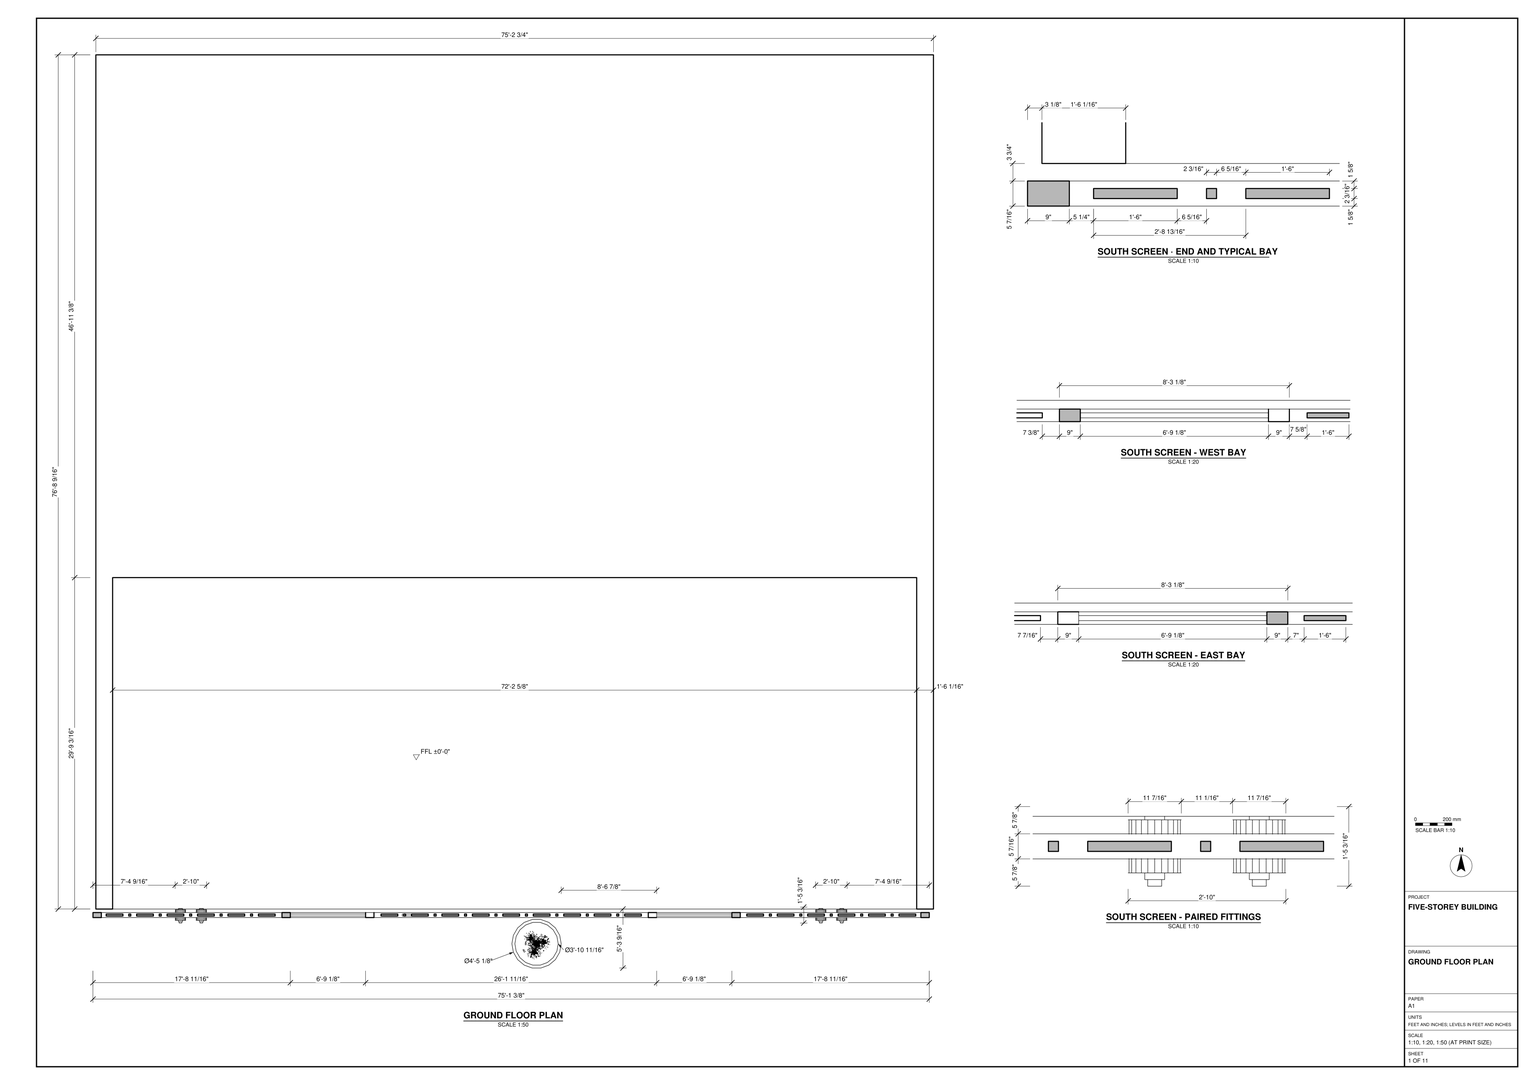
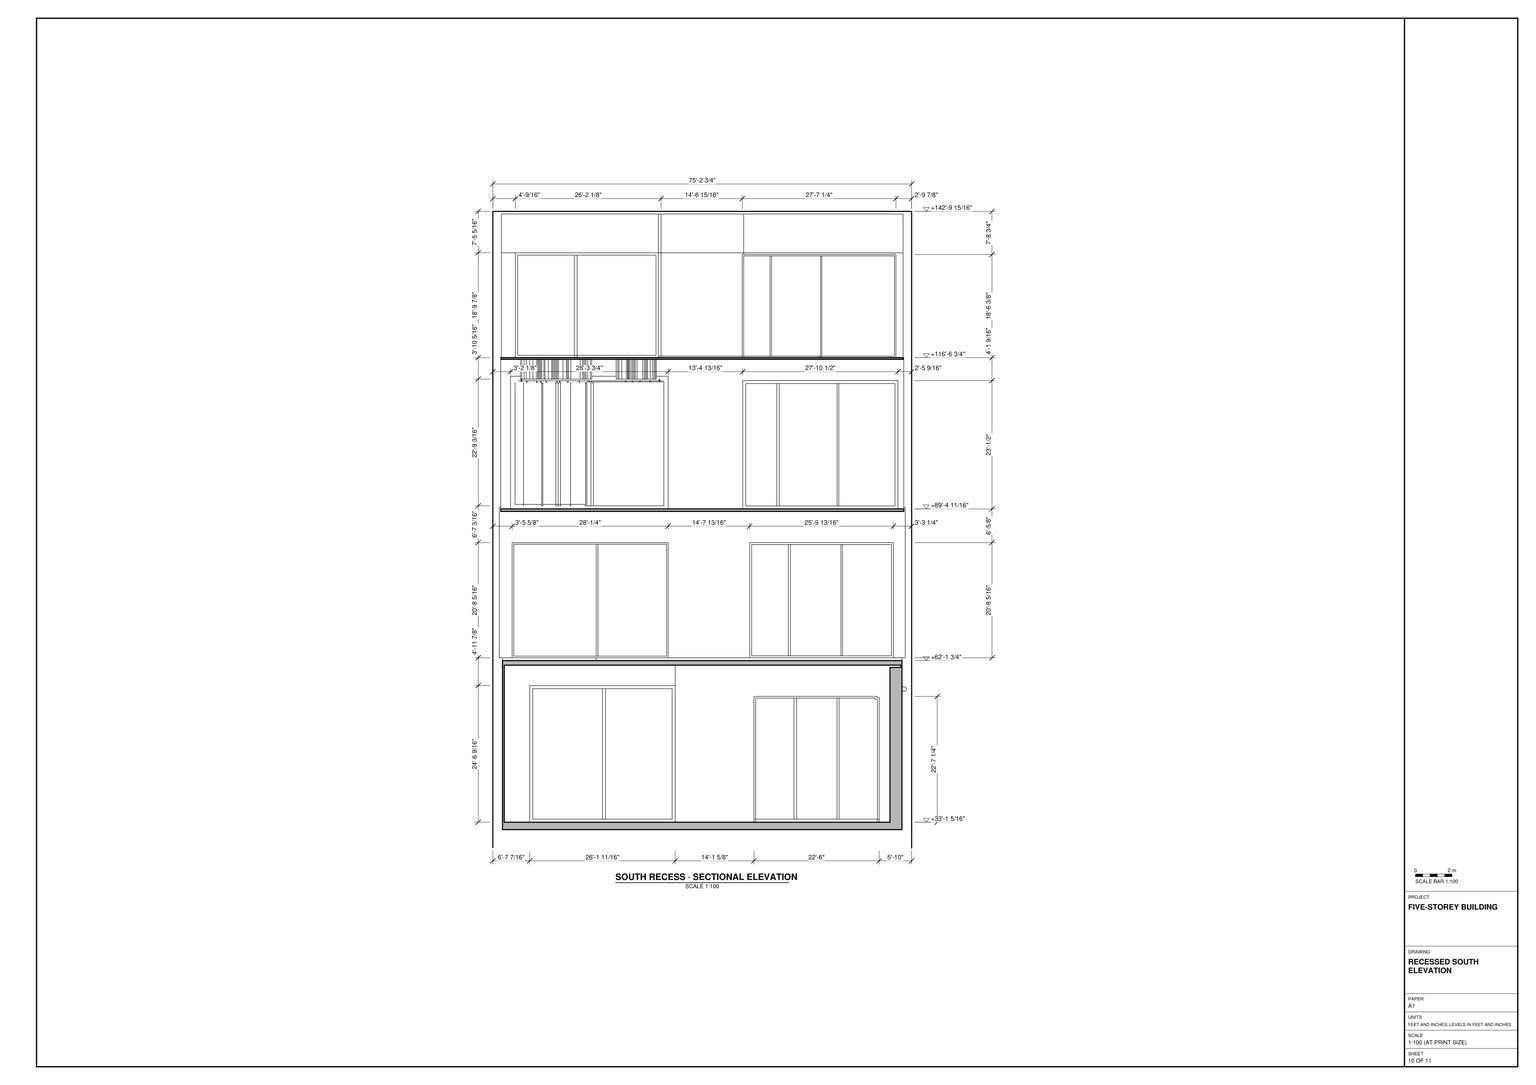
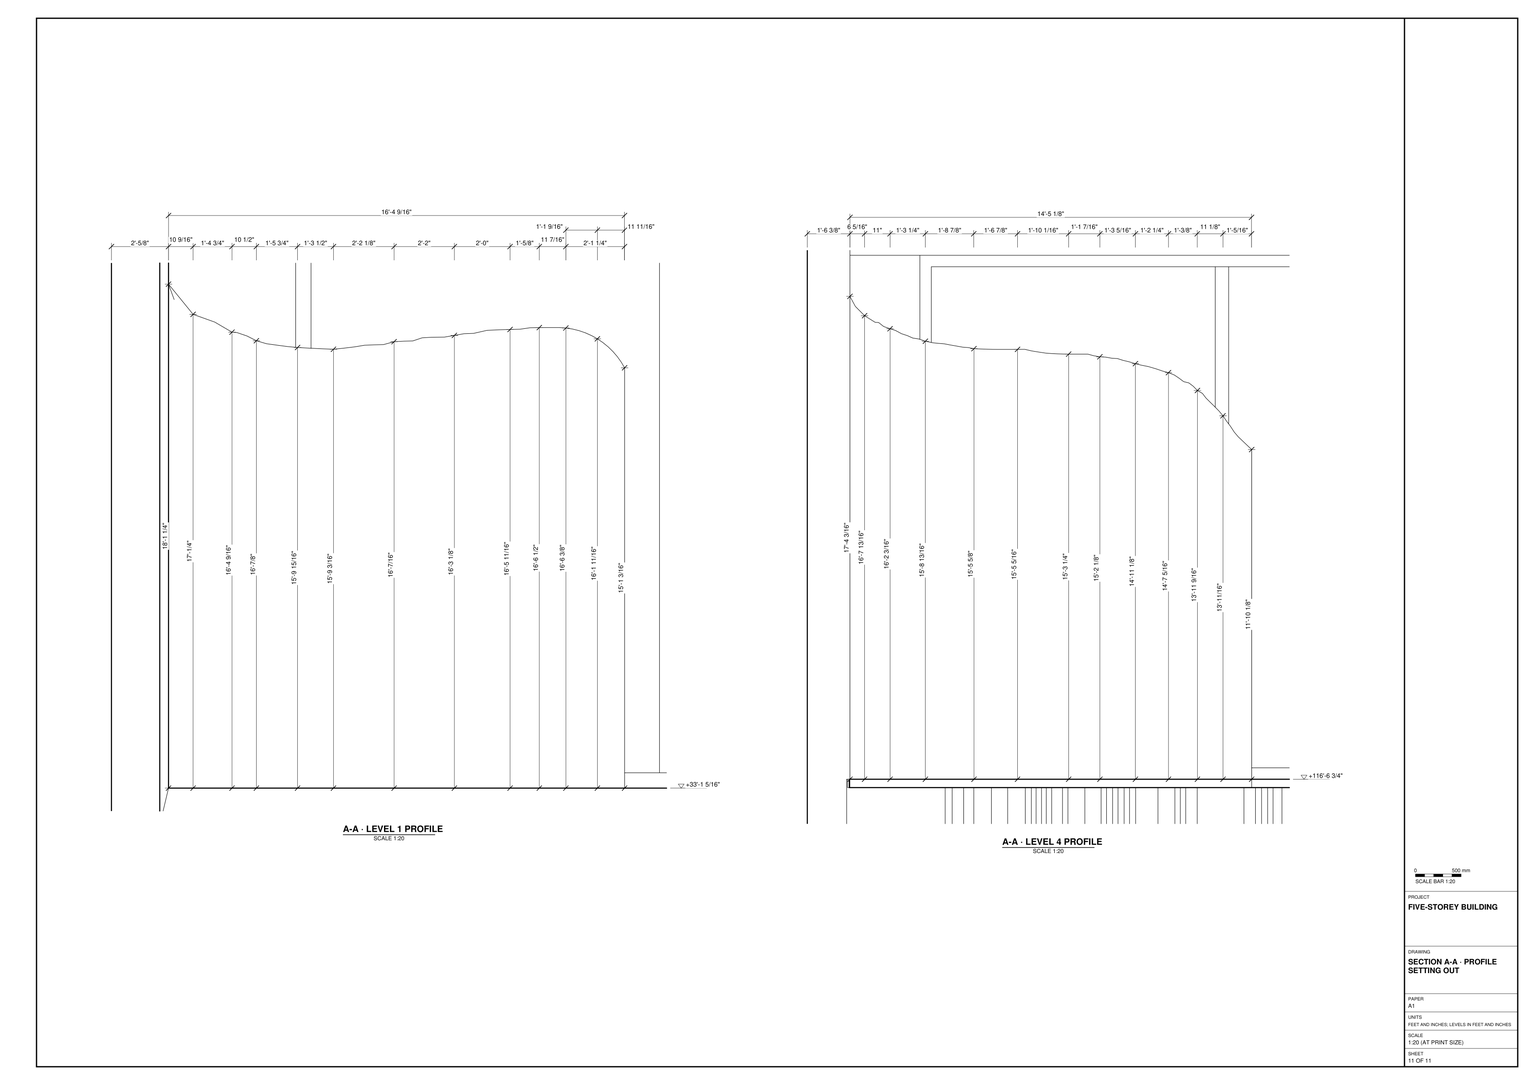
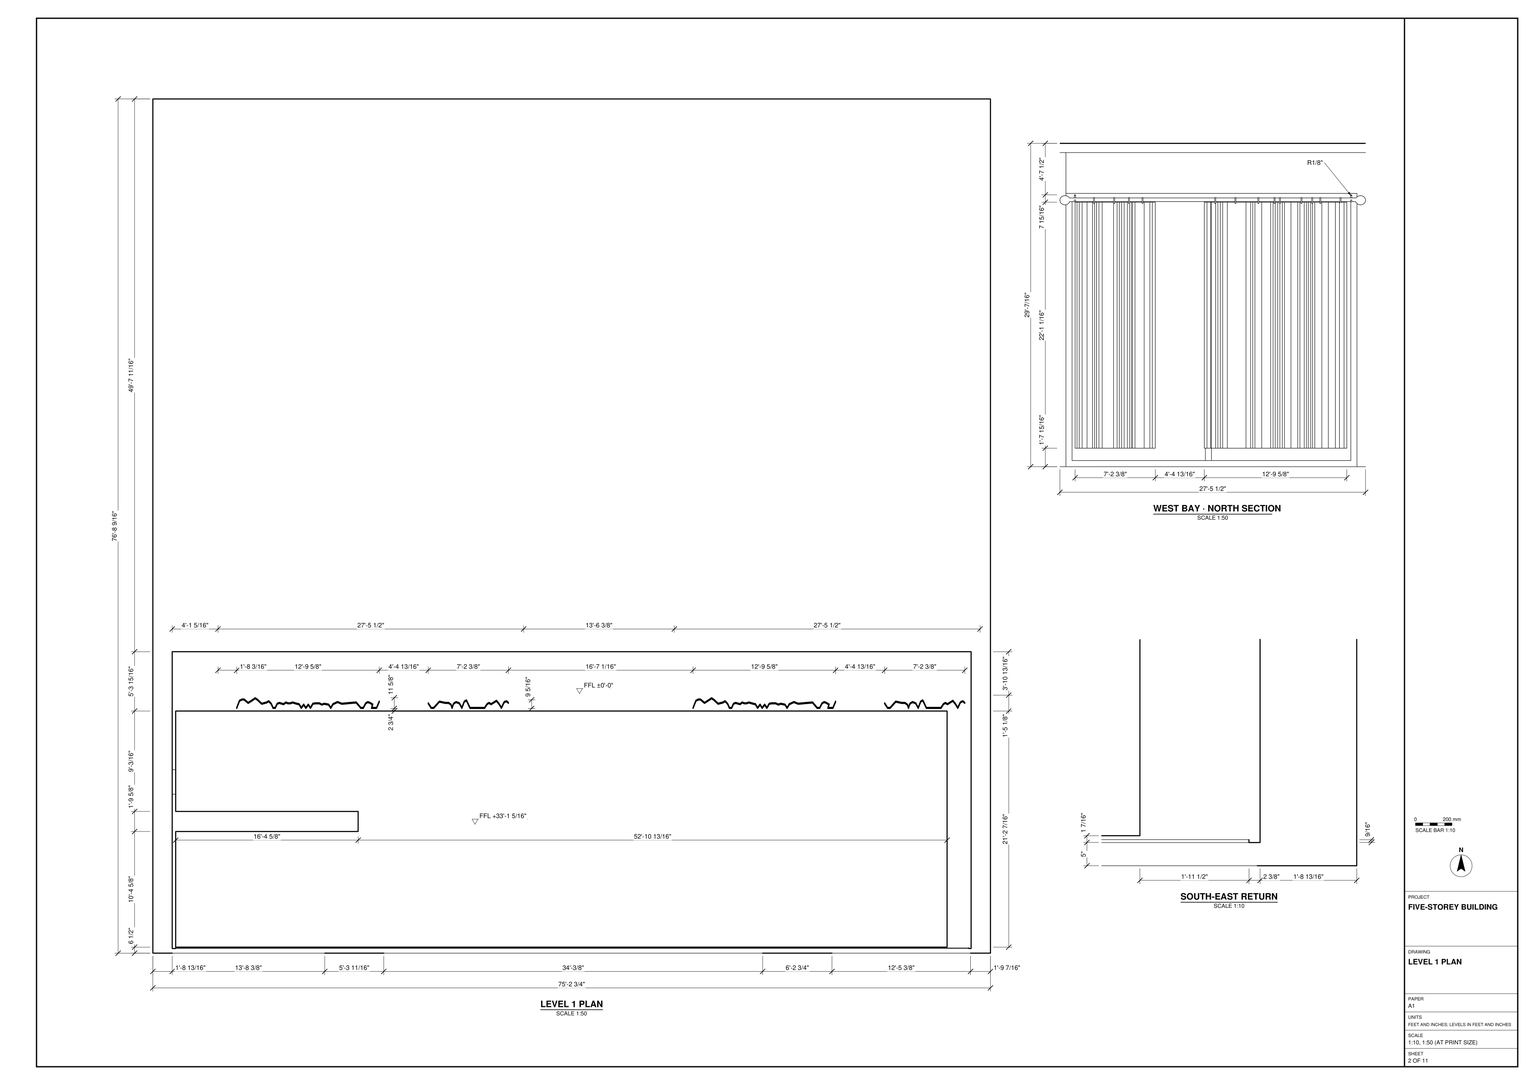
Build the five-storey building and its site in SketchUp from task_files/diagram_01.pdf. Work in feet and inches. The complete model, including the site, measures 266'-2 1/16" along X, 790'-1 5/16" along Y and 212'-3 1/8" along Z. Use the plans to size the building footprint rather than treating the overall model extents as wall dimensions. Set the floor levels to ±0'-0", +33'-1 5/16", +62'-1 3/4", +89'-4 11/16" and +116'-6 3/4".

Build the walls at their drawn thicknesses, with the floor slabs, roof and openings positioned from the plans and sections. Follow the sheets for any stairs, built-in joinery and main furniture shown. At ground level, model the south screen across the frontage, including its end posts, bay divisions and paired fittings. Place the plant outside the screen as shown in plan. Decor and loose items may use any suitable library component.

Above the screen, set the framed openings back into the south recess. Follow the sectional elevation for the widths, heads and panel divisions of the left and right openings on each floor. Use the setting-out heights in section A-A to shape the distinct profiles at levels 1 and 4. Keep shell elements such as walls, slabs and roof, and each furniture or joinery piece, in separate groups or components. Use components for repeated parts. Save one SketchUp model as output_files/five_storey_building_with_its_recessed_south_elevation.skp.

# SketchUp Ruby script. Lengths in inches.
U = 1.inch
M = Sketchup.active_model
def pt(a) = Geom::Point3d.new(a.map { |v| v * U })
def face(e, loops, mat)
  f = e.add_face(loops[0].map { |a| pt(a) })
  loops[1..].each { |l| e.add_face(l.map { |a| pt(a) }).erase! }
  f.material = f.back_material = mat if mat
  f
end
# faces: each face lists its corners as indices into pts; further lists are holes
def faces(e, pts, list, mat = nil) = list.each { |f| face(e, (f[0].is_a?(Array) ? f : [f]).map { |l| l.map { |i| pts[i] } }, mat) }
# xy, xz, yz: faces in a plane at the given z, y or x. An outline is a flat list of corners, or four numbers for a rectangle; further outlines are holes
def ring(l) = l.size == 4 ? [[l[0], l[1]], [l[2], l[1]], [l[2], l[3]], [l[0], l[3]]] : l.each_slice(2).to_a
def flat(e, list, mat, &to3) = list.each { |f| face(e, (f[0].is_a?(Array) ? f : [f]).map { |l| ring(l).map { |u, v| to3.(u, v) } }, mat) }
def xy(e, z, list, mat = nil) = flat(e, list, mat) { |x, y| [x, y, z] }
def xz(e, y, list, mat = nil) = flat(e, list, mat) { |x, z| [x, y, z] }
def yz(e, x, list, mat = nil) = flat(e, list, mat) { |y, z| [x, y, z] }
def lines(e, pts, list) = list.each { |a, b| e.add_line(pt(pts[a]), pt(pts[b])) }
# prism: a flat outline (further loops are holes) pulled along v
def prism(e, loops, v, mat = nil)
  f = face(e, loops, mat); d = Geom::Vector3d.new(v.map { |x| x * U })
  f.pushpull(f.normal.samedirection?(d) ? d.length : -d.length)
end
def box(e, o, s, mat = nil) = prism(e, [[o, [o[0] + s[0], o[1], o[2]], [o[0] + s[0], o[1] + s[1], o[2]], [o[0], o[1] + s[1], o[2]]]], [0, 0, s[2]], mat)
def at(x, y, z, deg = 0) = Geom::Transformation.translation(pt([x, y, z])) * Geom::Transformation.rotation(ORIGIN, Z_AXIS, deg.degrees)
def axes(o, x, y, z) = Geom::Transformation.new([*x, 0, *y, 0, *z, 0, *pt(o).to_a, 1])
def part(name) = M.definitions.add(name)
# library, detail: a bought-in or finely detailed component or shape, given as its bounding box
def library(name, o, s) = part(name).tap { |d| box(d.entities, o, s) }
def detail(e, o, s) = box(e.add_group.entities, o, s)
def put(e, d, t, mat = nil) = e.add_instance(d, t).tap { |i| i.material = mat if mat }
def group(e, t, mat = nil) = e.add_group.tap { |g| g.transformation = t; g.material = mat if mat }.entities
root = M.entities
M.materials.add("[0010_Snow]").color = [255, 250, 250]
M.materials.add("[0012_Bisque]").color = [255, 228, 196]
M.materials.add("[Aluminum]").color = [179, 179, 179]
M.materials.add("[Asphalt New]").color = [67, 60, 62]
M.materials.add("[Grass Dark Green]").color = [106, 157, 55]
M.materials.add("[Polished Concrete New]").color = [200, 200, 203]
M.materials.add("[Translucent Glass Gray]").color = [128, 128, 128]
M.materials["[Translucent Glass Gray]"].alpha = 0.5
c1 = library("ss",[-5.48,-0.48,0],[89.34,2.96,81.1])
c2 = library("Gate (1)",[0,0,0],[196.8,3.75,63.1])
c3 = library("plant_176_fbx.FBX\#1",[-22.43,-22.29,0],[44.86,44.58,89.56])
c4 = part("plant")
put(c4.entities,c3,axes([-2080.28,-4593.05,-0.53],[3.35,0,0],[0,3.35,0],[0,0,3.35]))
put(c4.entities,c3,at(-982.17,-787.56,-815.125))
c5 = library("Omni Light\#4",[-12,-12,-12],[24,24,24])
xy(root,0,[[1420,2023.15,2322.75,2943.71]])
xy(root,0,[[0,0,3194.0625,9481.3125]],"[Grass Dark Green]")
xy(root,0,[[1420,1658.7,2322.75,2023.15]],"[Polished Concrete New]")
xy(root,18.06,[[1438.06,2023.15,2304.69,2380.34]])
xy(root,359.51,[[1438.06,2023.15,2304.69,2045.6875],[1438.06,2045.6875,2304.69,2380.34]])
xy(root,399.48,[[1440.83,2028.15,2301.92,2348.03]])
xy(root,415.38,[[1444.61,2028.15,2299.52,2028.78],[1444.61,2029.63,2276.02,2029.63,2276.02,2284.09,1444.61,2284.09,1444.61,2175.87,1641.23,2175.87,1641.23,2154.25,1444.61,2154.25]])
xy(root,502.5,[[1444.61,2028.78,2299.52,2029.63]])
xy(root,749.17,[[2276.02,2029.63,2299.52,2255.15]])
xy(root,753.93,[[1444.61,2028.15,2299.52,2284.09]])
xy(root,763.83,[[1440.83,2028.15,2301.92,2036.8],[1440.83,2038.01,2301.92,2038.01,2301.92,2320.78,1440.83,2320.78,1440.83,2162.46,1611.58,2162.46,1611.58,2140.29,1440.83,2140.29]])
xy(root,769.83,[[1440.83,2320.78,1642.8,2348.03],[1642.8,2320.78,2301.92,2348.03]])
xy(root,862.14,[[1440.83,2036.8,2301.92,2038.01]])
xy(root,985.14,[[1440.83,2140.29,1526.21,2162.46]])
xy(root,1085.39,[[1436.97,2030.09,2305.78,2307.53]])
xy(root,1090.76,[[1436.97,2030.09,2305.78,2041.52],[1436.97,2042.7,2305.78,2042.7,2305.78,2285.9,1436.97,2285.9,1436.97,2160.46,1611.58,2160.46,1611.58,2140.29,1436.97,2140.29]])
xy(root,1176.39,[[1436.97,2041.52,2305.78,2042.7]])
xy(root,1299.33,[[1436.97,2140.29,1563.07,2160.46]])
xy(root,1413.24,[[1438.73,2020.1875,1438.38,2081.72,1438.38,2140.29,1611.58,2140.29,1611.58,2152.66,1438.38,2152.66,1438.38,2263.82,2304.37,2268.78,2304.37,2025.14,1956.49,2023.15],[2304.37,2025.14,2304.37,2268.78,2305.76,2025.15],[1438.38,2081.72,1437.34,2263.8125,1438.38,2263.82,1438.38,2152.66,1611.58,2152.66,1611.58,2140.29,1438.38,2140.29]])
xy(root,1416.84,[[1438.73,2020.1875,2305.76,2025.15,2305.76,2025.92,1438.73,2020.96],[1438.72,2021.46,2305.76,2026.42,2304.37,2268.78,2288.85,2268.6875,2126.46,2267.76,2123.22,2267.74,1957.59,2266.79,1776.75,2265.76,1601.67,2264.75,1595.88,2264.72,1468.55,2263.99,1437.34,2263.8125]])
xy(root,1487.46,[[1438.73,2020.96,2305.76,2025.92,2305.76,2026.42,1438.72,2021.46]])
xy(root,1600.09,[[1535.71,2140.29,1538.18,2152.66]])
xy(root,1602.13,[[1502.27,2140.29,1505.3125,2152.66]])
xy(root,1732,[[1420,2023.15,2322.75,2943.71]])
xz(root,2023.15,[[1686.8,415.06,1692.78,415.38,1684.8125,415.38],[1664.87,457.77,1669.95,463.91,1665.88,459.51],[1836.06,664.62,1841.67,671.4,1840.35,670.17],[1907.2,664.89,1902.87,670.41,1901.54,671.63]])
xz(root,2023.15,[[1420,0,2322.75,0,2322.75,378.65,2304.69,378.65,2304.69,18.06,1438.06,18.06,1438.06,378.65,1420,378.65],[[1438.06,359.51,2304.69,359.51,2304.69,378.65,2322.75,378.65,2322.75,726.9,1420,726.9,1420,378.65,1438.06,378.65],[1458.29,415.06,1456.01,415.2,1453.77,415.65,1451.61,416.38,1449.56,417.39,1447.66,418.66,1445.95,420.17,1444.44,421.88,1443.17,423.78,1442.16,425.83,1441.43,427.99,1440.98,430.23,1440.83,432.51,1440.83,679.94,1441.07,683.53,1441.77,687.07,1442.93,690.48,1444.52,693.71,1446.52,696.7,1448.9,699.41,1451.61,701.78,1454.6,703.78,1457.83,705.38,1461.24,706.54,1464.77,707.24,1468.37,707.47,1739.61,707.47,1746.38,706.83,1752.92,704.91,1758.97,701.78,1764.32,697.57,1768.77,692.42,1772.17,686.52,1774.39,680.08,1775.36,673.34,1775.02,666.54,1773.41,659.93,1770.57,653.74,1766.61,648.2,1563.8125,415.06],[1686.8,415.06,1684.8125,415.38,1680.875,416.02,1675.3,418.23,1670.32,421.58,1666.18,425.91,1663.06,431.03,1661.1,436.7,1660.41,442.66,1661,448.63,1662.85,454.33,1664.87,457.77,1665.88,459.51,1669.95,463.91,1836.06,664.62,1840.35,670.17,1841.67,671.4,1845.49,674.95,1851.35,678.81,1857.77,681.65,1864.57,683.4,1871.56,684,1878.55,683.45,1885.36,681.75,1891.8,678.96,1897.6875,675.14,1901.54,671.63,1902.87,670.41,1907.2,664.89,2078.61,460.9375,2079.75,459.14,2082.07,452.68,2082.9,445.88,2082.2,439.06,2080.01,432.56,2076.45,426.71,2071.67,421.79,2065.93,418.04,2059.5,415.66,2057.39,415.38,1692.78,415.38],[2226.625,424.75,2212.05,425.9,2197.83,429.34,2184.33,434.96,2171.875,442.64,2160.79,452.17,2151.34,463.34,2004.24,667.8,2003.55,670.71,2003.23,673.67,2003.31,676.66,2003.76,679.61,2004.59,682.47,2005.77,685.21,2007.3,687.77,2009.15,690.12,2011.28,692.21,2013.66,694.01,2016.25,695.49,2019.01,696.625,2258.35,696.625,2264.04,696.25,2269.625,695.14,2275.02,693.31,2280.13,690.79,2284.87,687.62,2289.16,683.86,2292.91,679.58,2296.08,674.84,2298.6,669.73,2300.43,664.33,2301.54,658.75,2301.92,653.06,2301.92,463.34,2292.47,452.17,2281.38,442.64,2268.93,434.96,2255.43,429.34,2241.21,425.9]],[1420,726.9,2322.75,756.05],[[1420,756.05,2322.75,1079.67],[1688.07,769.83,1571.26,998.05,1571.0625,1001.98,1571.41,1005.91,1572.32,1009.74,1573.75,1013.41,1575.68,1016.84,1578.08,1019.97,1580.89,1022.73,1584.0625,1025.06,1587.53,1026.93,1591.23,1028.29,1595.08,1029.12,1599.01,1029.4,1915.93,1029.4,2050.45,832.63,2055.45,827.41,2059.28,821.29,2060.58,817.82,2061.8125,814.52,2062.92,807.375,2062.57,800.16,2060.77,793.16,2057.6,786.67,2053.18,780.95,2047.7,776.24,2041.38,772.72,2034.49,770.56,2027.3,769.83],[2244.03,769.83,2038.48,1013.54,2037.45,1015.04,2036.71,1016.7,2036.3,1018.48,2036.23,1020.3,2036.5,1022.1,2037.11,1023.82,2038.03,1025.39,2039.23,1026.76,2040.67,1027.88,2042.29,1028.71,2044.04,1029.22,2045.85,1029.4,2286.62,1029.4,2289.53,1029.21,2292.4,1028.63,2295.17,1027.69,2297.79,1026.4,2300.23,1024.78,2302.42,1022.85,2304.35,1020.65,2305.98,1018.22,2307.27,1015.6,2308.21,1012.83,2308.78,1009.96,2308.97,1007.04,2308.97,803.58,2305.13,798.54,2300.89,793.83,2296.29,789.47,2291.36,785.49,2286.13,781.91,2280.625,778.77,2274.89,776.07,2268.96,773.84,2262.87,772.09,2256.65,770.84,2250.36,770.08],[1484.19,769.83,1482.23,771.84,1480.4,773.99,1478.73,776.25,1477.2,778.61,1475.84,781.08,1474.65,783.63,1473.64,786.25,1472.8,788.94,1472.14,791.68,1471.67,794.45,1471.39,797.25,1471.3,800.07,1471.3,976.54,1475.75,981.75,1480.95,986.19,1486.79,989.77,1493.12,992.38,1499.77,993.98,1506.6,994.52,1513.42,993.98,1520.08,992.38,1526.41,989.77,1532.25,986.19,1537.45,981.75,1541.9,976.54,1635.43,784.92,1636.07,783.27,1636.42,781.54,1636.48,779.77,1636.24,778.02,1635.71,776.33,1634.9,774.76,1633.84,773.34,1632.56,772.13,1631.09,771.14,1629.48,770.42,1627.77,769.98,1626,769.83]],[[1420,1079.67,2322.75,1394.86],[1680.57,1107.14,1571.26,1320.7,1571.0625,1324.64,1571.41,1328.56,1572.32,1332.39,1573.75,1336.06,1575.68,1339.5,1578.08,1342.625,1580.89,1345.38,1584.0625,1347.72,1587.53,1349.58,1591.23,1350.95,1595.08,1351.77,1599.01,1352.05,1915.93,1352.05,2050.45,1155.29,2055.45,1150.0625,2059.28,1143.94,2060.58,1140.47,2061.8125,1137.17,2062.92,1130.03,2062.57,1122.8125,2060.77,1115.8125,2057.6,1109.32,2055.91,1107.14],[2244.03,1092.48,2038.48,1336.19,2037.45,1337.6875,2036.71,1339.36,2036.3,1341.13,2036.23,1342.95,2036.5,1344.75,2037.11,1346.47,2038.03,1348.04,2039.23,1349.42,2040.67,1350.54,2042.29,1351.37,2044.04,1351.88,2045.85,1352.05,2286.62,1352.05,2289.53,1351.86,2292.4,1351.29,2295.17,1350.35,2297.79,1349.06,2300.23,1347.43,2302.42,1345.5,2304.35,1343.3,2305.78,1341.17,2305.98,1340.87,2307.27,1338.25,2308.21,1335.48,2308.78,1332.61,2308.97,1329.69,2308.97,1126.23,2305.78,1122.05,2305.13,1121.2,2300.89,1116.48,2296.29,1112.12,2291.36,1108.14,2289.89,1107.14,2286.13,1104.57,2280.625,1101.42,2274.89,1098.73,2269.33,1096.64,2268.96,1096.5,2262.87,1094.75,2256.65,1093.49,2250.36,1092.73],[1484.19,1092.48,1482.23,1094.5,1480.4,1096.64,1478.73,1098.9,1477.2,1101.27,1475.84,1103.73,1474.65,1106.28,1474.32,1107.14,1473.64,1108.91,1472.8,1111.59,1472.14,1114.33,1471.67,1117.11,1471.39,1119.91,1471.3,1122.72,1471.3,1299.2,1475.75,1304.4,1480.95,1308.84,1486.79,1312.42,1493.12,1315.04,1499.77,1316.63,1506.6,1317.17,1513.42,1316.63,1520.08,1315.04,1526.41,1312.42,1532.25,1308.84,1537.45,1304.4,1541.9,1299.2,1635.43,1107.58,1635.6,1107.14,1636.07,1105.93,1636.42,1104.19,1636.48,1102.43,1636.24,1100.67,1635.71,1098.99,1634.9,1097.41,1634.32,1096.64,1633.84,1096,1632.56,1094.78,1631.09,1093.8,1629.48,1093.07,1627.77,1092.63,1626,1092.48]],
  [[1420,1394.86,2322.75,1732],[1491.65,1413.24,1484.69,1413.69,1477.86,1415.05,1471.26,1417.29,1465.01,1420.37,1459.22,1424.24,1453.98,1428.84,1449.39,1434.07,1445.52,1439.87,1442.43,1446.12,1440.19,1452.71,1438.84,1459.55,1438.38,1466.5,1438.38,1587.1,1438.86,1594.46,1440.3,1601.7,1442.67,1608.68,1445.93,1615.29,1450.03,1621.43,1454.89,1626.97,1460.4375,1631.83,1466.57,1635.93,1473.19,1639.19,1480.17,1641.5625,1487.4,1643,1494.76,1643.49,1904.25,1643.49,2121.47,1466.5,2121.26,1459.625,2120.13,1452.84,2118.11,1446.27,2115.23,1440.02,2111.54,1434.22,2107.11,1428.96,2102.02,1424.34,2096.35,1420.4375,2090.21,1417.33,2083.72,1415.07,2076.98,1413.7,2070.11,1413.24],[2285.24,1461.85,2282.05,1462.03,2278.91,1462.57,2275.85,1463.47,2272.91,1464.71,2270.125,1466.27,2267.54,1468.13,2080.05,1620.43,2078.28,1621.86,2076.77,1623.56,2075.56,1625.48,2074.67,1627.56,2074.12,1629.77,2073.9375,1632.03,2074.12,1634.3,2074.67,1636.5,2075.56,1638.59,2076.77,1640.51,2078.28,1642.21,2080.05,1643.64,2283.92,1643.64,2286.59,1643.46,2289.21,1642.94,2291.74,1642.08,2294.14,1640.9,2296.37,1639.41,2298.38,1637.65,2300.14,1635.64,2301.63,1633.41,2302.8125,1631.01,2303.67,1628.48,2304.19,1625.85,2304.37,1623.18,2304.37,1490.32,2302.93,1468.13,2300.35,1466.27,2297.57,1464.71,2294.625,1463.47,2291.56,1462.57,2288.42,1462.03]]],"[0012_Bisque]")
xz(root,2028.15,[[[1440.83,399.48,2301.92,763.83],[1444.61,415.38,2299.52,753.93]]],"[Aluminum]")
xz(root,2029.63,[[2276.02,502.5,2299.52,749.17]],"[Aluminum]")
xz(root,2029.63,[[1444.61,415.38,2276.02,502.5]],"[Translucent Glass Gray]")
xz(root,2030.09,[[1436.97,1085.39,2305.78,1090.76]])
xz(root,2038.01,[[1440.83,763.83,2301.92,862.14]],"[Translucent Glass Gray]")
xz(root,2042.7,[[1436.97,1090.76,2305.78,1176.39]],"[Translucent Glass Gray]")
xz(root,2140.29,[[1440.83,763.83,1611.58,763.83,1611.58,935.09,1607.03,942.44,1601.85,949.36,1596.08,955.79,1589.76,961.69,1582.94,967.01,1575.6875,971.71,1568.05,975.74,1560.08,979.09,1551.84,981.72,1543.41,983.61,1534.84,984.76,1526.21,985.14,1440.83,985.14],[1436.97,1090.76,1611.58,1090.76,1611.58,1250.82,1611.17,1257.15,1609.93,1263.375,1607.89,1269.38,1605.08,1275.07,1601.56,1280.35,1597.375,1285.12,1592.6,1289.3,1587.33,1292.83,1581.64,1295.64,1575.63,1297.67,1569.41,1298.91,1563.07,1299.33,1436.97,1299.33],[1438.38,1413.24,1611.58,1413.24,1611.58,1558.95,1605.79,1564.46,1604.09,1566.46,1602.37,1569.08,1600.65,1571.33,1599.2,1573.53,1597.4,1575.67,1595.34,1577.76,1593.59,1579.46,1591.85,1581.2,1590.35,1583.16,1588.2,1584.41,1586.36,1586.28,1584.48,1587.7,1582.26,1588.23,1580.3,1589.71,1578.22,1591.11,1575.71,1592.125,1573.13,1592.81,1570.22,1593.8,1567,1594.75,1563.92,1595.35,1561.47,1595.99,1558.46,1596.86,1556.1,1597.41,1553.72,1598.1875,1551.29,1598.33,1548.57,1598.81,1546.13,1598.96,1543.4,1599.42,1540.92,1600.1,1538.18,1600.09,1535.71,1600.09,1532.68,1600.1,1530.31,1600.14,1527.85,1600.22,1525.34,1600.34,1522.75,1600.54,1519.51,1601.03,1516.65,1601.49,1513.77,1602.17,1510.62,1602.15,1508.13,1602.14,1505.3125,1602.13,1502.27,1602.13,1499.85,1602.16,1497.42,1602.22,1494.9375,1602.31,1491.86,1602.45,1489.44,1602.92,1486.99,1603.1,1484.23,1603.6,1481.51,1604.07,1479.0625,1604.54,1476.58,1604.74,1474.02,1605,1470.89,1605.67,1468.15,1606.62,1465.43,1607.04,1463.07,1608.1,1460.65,1608.89,1457.97,1610.33,1455.67,1611.04,1452.91,1612.01,1450.73,1613.74,1449.29,1613.79,1444.7,1616.65,1440.72,1620.66,1438.38,1624.99]],"[0012_Bisque]")
xz(root,2152.66,[[1438.38,1413.24,1438.38,1624.99,1440.72,1620.66,1444.7,1616.65,1449.29,1613.79,1450.73,1613.74,1452.91,1612.01,1455.67,1611.04,1457.97,1610.33,1460.65,1608.89,1463.07,1608.1,1465.43,1607.04,1468.15,1606.62,1470.89,1605.67,1474.02,1605,1476.58,1604.74,1479.0625,1604.54,1481.51,1604.07,1484.23,1603.6,1486.99,1603.1,1489.44,1602.92,1491.86,1602.45,1494.9375,1602.31,1497.42,1602.22,1499.85,1602.16,1502.27,1602.13,1505.3125,1602.13,1508.13,1602.14,1510.62,1602.15,1513.77,1602.17,1516.65,1601.49,1519.51,1601.03,1522.75,1600.54,1525.34,1600.34,1527.85,1600.22,1530.31,1600.14,1532.68,1600.1,1535.71,1600.09,1538.18,1600.09,1540.92,1600.1,1543.4,1599.42,1546.13,1598.96,1548.57,1598.81,1551.29,1598.33,1553.72,1598.1875,1556.1,1597.41,1558.46,1596.86,1561.47,1595.99,1563.92,1595.35,1567,1594.75,1570.22,1593.8,1573.13,1592.81,1575.71,1592.125,1578.22,1591.11,1580.3,1589.71,1582.26,1588.23,1584.48,1587.7,1586.36,1586.28,1588.2,1584.41,1590.35,1583.16,1591.85,1581.2,1593.59,1579.46,1595.34,1577.76,1597.4,1575.67,1599.2,1573.53,1600.65,1571.33,1602.37,1569.08,1604.09,1566.46,1605.79,1564.46,1611.58,1558.95,1611.58,1413.24]])
xz(root,2154.25,[[1444.61,415.38,1641.23,415.38,1641.23,596.56,1639.76,599.05,1638.07,601.4,1636.1875,603.6,1634.12,605.62,1631.87,607.45,1629.48,609.07,1626.95,610.47,1624.3,611.65,1621.5625,612.59,1618.75,613.28,1615.89,613.73,1613.01,613.91,1608.46,613.92,1604.45,613.9,1600.4,613.82,1596.1875,613.21,1591.84,613.09,1587.42,612.96,1581.93,612.71,1576.14,611.41,1571.99,611.25,1567.82,610.53,1563.55,609.8,1557.89,609.73,1553.95,609.49,1549.91,608.15,1545.92,608.04,1541.86,607.83,1537.27,606.5625,1533.23,606.47,1529.14,606.29,1524.9,605.6,1520.08,605.02,1515.7,604.5625,1510.8,604.77,1505.46,605.02,1500.24,605.32,1496.14,605.7,1491.96,606.24,1486.8,606.95,1482.49,608.23,1478.43,610.28,1474.07,611.77,1471.96,611.9375,1464.56,616.26,1455.21,619.61,1444.61,632.63]],"[0012_Bisque]")
xz(root,2160.46,[[1436.97,1090.76,1436.97,1299.33,1563.07,1299.33,1569.41,1298.91,1575.63,1297.67,1581.64,1295.64,1587.33,1292.83,1592.6,1289.3,1597.375,1285.12,1601.56,1280.35,1605.08,1275.07,1607.89,1269.38,1609.93,1263.375,1611.17,1257.15,1611.58,1250.82,1611.58,1090.76]])
xz(root,2162.46,[[1440.83,763.83,1440.83,985.14,1526.21,985.14,1534.84,984.76,1543.41,983.61,1551.84,981.72,1560.08,979.09,1568.05,975.74,1575.6875,971.71,1582.94,967.01,1589.76,961.69,1596.08,955.79,1601.85,949.36,1607.03,942.44,1611.58,935.09,1611.58,763.83]])
xz(root,2175.87,[[1444.61,415.38,1444.61,632.63,1455.21,619.61,1464.56,616.26,1471.96,611.9375,1474.07,611.77,1478.43,610.28,1482.49,608.23,1486.8,606.95,1491.96,606.24,1496.14,605.7,1500.24,605.32,1505.46,605.02,1510.8,604.77,1515.7,604.5625,1520.08,605.02,1524.9,605.6,1529.14,606.29,1533.23,606.47,1537.27,606.5625,1541.86,607.83,1545.92,608.04,1549.91,608.15,1553.95,609.49,1557.89,609.73,1563.55,609.8,1567.82,610.53,1571.99,611.25,1576.14,611.41,1581.93,612.71,1587.42,612.96,1591.84,613.09,1596.1875,613.21,1600.4,613.82,1604.45,613.9,1608.46,613.92,1613.01,613.91,1615.89,613.73,1618.75,613.28,1621.5625,612.59,1624.3,611.65,1626.95,610.47,1629.48,609.07,1631.87,607.45,1634.12,605.62,1636.1875,603.6,1638.07,601.4,1639.76,599.05,1641.23,596.56,1641.23,415.38]])
xz(root,2268.78,[[1438.38,1642.7,1776.73,1726.37],[1782.64,1642.7,2304.37,1726.37]],"[Polished Concrete New]")
xz(root,2268.78,[[1438.38,1413.24,2304.37,1642.7],[1776.73,1642.7,1782.64,1726.37]],"[Translucent Glass Gray]")
xz(root,2284.09,[[1444.61,415.38,1499.43,415.38,1499.43,709.94,1813.12,709.94,1813.12,753.93,1444.61,753.93]],"[Aluminum]")
xz(root,2284.09,[[[1499.43,415.38,1813.12,709.94],[1506.04,421.99,1806.5,703.33]],[1982.74,415.38,1986.52,421.99],[1986.52,415.38,2248.95,421.99],[2248.95,415.38,2252.72,421.99],[1656.27,421.99,1662.79,703.33],
  [1982.74,421.99,1986.52,421.99,1986.52,682.87,2243.81,682.87,2243.81,680.73,2248.95,680.73,2248.95,421.99,2252.72,421.99,2252.72,684.51,2247.58,684.51,2247.58,686.64,1982.74,686.64],[2069.07,421.99,2074.82,682.87],[2161.88,421.99,2166.39,682.87]],"[Asphalt New]")
xz(root,2284.09,[[1813.12,415.38,1982.74,415.38,1982.74,686.64,2247.58,686.64,2247.58,684.51,2252.72,684.51,2252.72,415.38,2276.02,415.38,2276.02,720.22,2299.52,720.22,2299.52,753.93,1813.12,753.93]],"[Polished Concrete New]")
xz(root,2284.09,[[1506.04,421.99,1656.27,703.33],[1662.79,421.99,1806.5,703.33],[1986.52,421.99,2069.07,682.87],[2074.82,421.99,2161.88,682.87],[2166.39,421.99,2248.95,421.99,2248.95,680.73,2243.81,680.73,2243.81,682.87,2166.39,682.87]],"[Translucent Glass Gray]")
xz(root,2285.9,[[[1458.125,1090.76,1797.875,1376.64],[1467.93,1100.58,1788.0625,1366.83]],[[1958.71,1090.76,2293.21,1367.26],[1965.05,1097.11,2286.87,1360.92]],[2032.16,1097.11,2037.37,1360.92],[2162.12,1097.11,2165.71,1360.92],[1628,1100.58,1632.72,1366.83]],"[Asphalt New]")
xz(root,2285.9,[[1436.97,1090.76,1458.125,1090.76,1458.125,1376.64,1797.875,1376.64,1797.875,1090.76,1958.71,1090.76,1958.71,1367.26,2293.21,1367.26,2293.21,1090.76,2305.78,1090.76,2305.78,1416.84,1436.97,1416.84]],"[Polished Concrete New]")
xz(root,2285.9,[[1965.05,1097.11,2032.16,1360.92],[2037.37,1097.11,2162.12,1360.92],[2165.71,1097.11,2286.87,1360.92],[1467.93,1100.58,1628,1366.83]],"[Translucent Glass Gray]")
xz(root,2307.53,[[1436.97,1085.39,2305.78,1107.14]])
xz(root,2320.78,[[1440.83,763.83,1642.8,769.83],[1642.8,763.83,2301.92,769.83]])
xz(root,2320.78,[[[1461.625,769.83,1797.875,1018.14],[1465.14,773.34,1794.36,1014.625]],[[1973.67,769.83,2283.49,1018.14],[1977.9,774.06,2279.26,1013.91]],[1642.8,773.34,1646.49,1014.625],[2056.98,774.06,2061.49,1013.91],[2170.375,774.06,2173.75,1013.91]],"[Asphalt New]")
xz(root,2320.78,[[1433.78,769.83,1461.625,769.83,1461.625,1018.14,1797.875,1018.14,1797.875,769.83,1973.67,769.83,1973.67,1018.14,2283.49,1018.14,2283.49,769.83,2308.97,769.83,2308.97,1094.04,1433.78,1094.04]],"[Polished Concrete New]")
xz(root,2320.78,[[1465.14,773.34,1642.8,1014.625],[1646.49,773.34,1794.36,1014.625],[1977.9,774.06,2056.98,1013.91],[2061.49,774.06,2170.375,1013.91],[2173.75,774.06,2279.26,1013.91]],"[Translucent Glass Gray]")
xz(root,2348.03,[[1440.83,399.48,2301.92,769.83]])
xz(root,2380.34,[[1438.06,18.06,2304.69,359.51]],"[0010_Snow]")
xz(root,2943.71,[[1420,0,2322.75,1732]])
yz(root,1420,[[2023.15,0,2943.71,1732]])
yz(root,1436.97,[[2030.09,1085.39,2030.09,1090.76,2041.52,1090.76,2041.52,1176.39,2042.7,1176.39,2042.7,1090.76,2140.29,1090.76,2140.29,1299.33,2160.46,1299.33,2160.46,1090.76,2285.9,1090.76,2285.9,1085.39],[2285.9,1085.39,2307.53,1107.14]])
yz(root,1438.06,[[2023.15,18.06,2380.34,359.51]])
yz(root,1440.83,[[2028.15,399.48,2028.15,763.83,2036.8,763.83,2036.8,862.14,2038.01,862.14,2038.01,763.83,2140.29,763.83,2140.29,769.83,2162.46,769.83,2162.46,763.83,2320.78,763.83,2320.78,769.83,2348.03,769.83,2348.03,399.48],[2140.29,769.83,2162.46,985.14]])
yz(root,1444.61,[[2028.15,415.38,2028.78,415.38,2028.78,502.5,2029.63,502.5,2029.63,415.38,2154.25,415.38,2154.25,632.63,2175.87,632.63,2175.87,415.38,2284.09,415.38,2284.09,753.93,2028.15,753.93]])
yz(root,1611.58,[[2140.29,763.83,2162.46,935.09],[2140.29,1090.76,2160.46,1250.82],[2140.29,1413.24,2152.66,1558.95]])
yz(root,1641.23,[[2154.25,415.38,2175.87,596.56]])
yz(root,2276.02,[[2029.63,415.38,2029.63,739.51,2051.08,742.45,2072.66,744.375,2094.29,745.27,2115.95,745.15,2137.58,744,2159.125,741.83,2180.54,738.65,2201.79,734.45,2222.82,729.26,2243.57,723.08,2264.01,715.92,2284.09,707.8,2284.09,415.38],[2284.09,707.8,2264.01,715.92,2243.57,723.08,2222.82,729.26,2201.79,734.45,2180.54,738.65,2159.125,741.83,2137.58,744,2115.95,745.15,2094.29,745.27,2072.66,744.375,2051.08,742.45,2029.63,739.51,2029.63,749.17,2255.15,749.17,2258.92,748.92,2262.64,748.18,2266.22,746.96,2269.62,745.29,2272.77,743.18,2275.61,740.6875,2278.11,737.84,2280.21,734.69,2281.89,731.3,2283.1,727.71,2283.84,724,2284.09,720.22],[2029.63,749.17,2051.04,749.46,2072.44,749.26,2075.34,749.17]])
yz(root,2299.52,[[2028.15,415.38,2028.15,753.93,2284.09,753.93,2284.09,720.22,2283.84,724,2283.1,727.71,2281.89,731.3,2280.21,734.69,2278.11,737.84,2275.61,740.6875,2272.77,743.18,2269.62,745.29,2266.22,746.96,2262.64,748.18,2258.92,748.92,2255.15,749.17,2029.63,749.17,2029.63,502.5,2028.78,502.5,2028.78,415.38]])
yz(root,2301.92,[[2028.15,399.48,2348.03,399.48,2348.03,769.83,2320.78,769.83,2320.78,763.83,2038.01,763.83,2038.01,862.14,2036.8,862.14,2036.8,763.83,2028.15,763.83]],"[Aluminum]")
yz(root,2304.69,[[2023.15,18.06,2380.34,359.51]])
yz(root,2305.78,[[2030.09,1085.39,2307.53,1085.39,2307.53,1107.14,2285.9,1107.14,2285.9,1090.76,2042.7,1090.76,2042.7,1176.39,2041.52,1176.39,2041.52,1090.76,2030.09,1090.76]])
yz(root,2322.75,[[2023.15,0,2943.71,1732]])
p = [[1440.83,2194.43,399.48],[1444.61,2194.43,415.38],[1444.61,2220.87,415.38],[1440.83,2220.87,399.48],[1639.76,2154.25,599.05],[1641.23,2154.25,596.56],
  [1641.23,2175.87,596.56],[1639.76,2175.87,599.05],[1638.07,2154.25,601.4],[1638.07,2175.87,601.4],[1636.1875,2154.25,603.6],[1636.1875,2175.87,603.6],
  [1634.12,2154.25,605.62],[1634.12,2175.87,605.62],[1510.8,2154.25,604.77],[1515.7,2154.25,604.5625],[1515.7,2175.87,604.5625],[1510.8,2175.87,604.77],
  [1520.08,2154.25,605.02],[1520.08,2175.87,605.02],[1505.46,2154.25,605.02],[1505.46,2175.87,605.02],[1500.24,2154.25,605.32],[1500.24,2175.87,605.32],
  [1524.9,2154.25,605.6],[1524.9,2175.87,605.6],[1496.14,2154.25,605.7],[1496.14,2175.87,605.7],[1529.14,2154.25,606.29],[1529.14,2175.87,606.29],
  [1631.87,2154.25,607.45],[1631.87,2175.87,607.45],[1491.96,2154.25,606.24],[1491.96,2175.87,606.24],[1486.8,2154.25,606.95],[1486.8,2175.87,606.95],
  [1533.23,2154.25,606.47],[1533.23,2175.87,606.47],[1537.27,2154.25,606.5625],[1537.27,2175.87,606.5625],[1541.86,2154.25,607.83],[1541.86,2175.87,607.83],
  [1482.49,2154.25,608.23],[1482.49,2175.87,608.23],[1629.48,2154.25,609.07],[1629.48,2175.87,609.07],[1545.92,2154.25,608.04],[1545.92,2175.87,608.04],
  [1549.91,2154.25,608.15],[1549.91,2175.87,608.15],[1553.95,2154.25,609.49],[1553.95,2175.87,609.49],[1478.43,2154.25,610.28],[1478.43,2175.87,610.28],
  [1626.95,2154.25,610.47],[1626.95,2175.87,610.47],[1557.89,2154.25,609.73],[1557.89,2175.87,609.73],[1563.55,2154.25,609.8],[1563.55,2175.87,609.8],
  [1567.82,2154.25,610.53],[1567.82,2175.87,610.53],[1474.07,2154.25,611.77],[1474.07,2175.87,611.77],[1571.99,2154.25,611.25],[1571.99,2175.87,611.25],
  [1624.3,2154.25,611.65],[1624.3,2175.87,611.65],[1576.14,2154.25,611.41],[1576.14,2175.87,611.41],[1581.93,2154.25,612.71],[1581.93,2175.87,612.71],
  [1621.5625,2154.25,612.59],[1621.5625,2175.87,612.59],[1471.96,2154.25,611.9375],[1471.96,2175.87,611.9375],[1464.56,2154.25,616.26],[1464.56,2175.87,616.26],
  [1618.75,2154.25,613.28],[1618.75,2175.87,613.28],[1587.42,2154.25,612.96],[1587.42,2175.87,612.96],[1591.84,2154.25,613.09],[1591.84,2175.87,613.09],
  [1596.1875,2154.25,613.21],[1596.1875,2175.87,613.21],[1600.4,2154.25,613.82],[1600.4,2175.87,613.82],[1615.89,2154.25,613.73],[1615.89,2175.87,613.73],
  [1613.01,2154.25,613.91],[1613.01,2175.87,613.91],[1604.45,2154.25,613.9],[1604.45,2175.87,613.9],[1608.46,2154.25,613.92],[1608.46,2175.87,613.92],
  [1455.21,2154.25,619.61],[1455.21,2175.87,619.61],[1444.61,2154.25,632.63],[1444.61,2175.87,632.63],[2299.52,2283.84,724],[2299.52,2284.09,720.22],
  [2276.02,2284.09,720.22],[2276.02,2283.84,724],[2299.52,2283.1,727.71],[2276.02,2283.1,727.71],[2299.52,2281.89,731.3],[2276.02,2281.89,731.3],
  [2299.52,2280.21,734.69],[2276.02,2280.21,734.69],[2299.52,2278.11,737.84],[2276.02,2278.11,737.84],[2299.52,2275.61,740.6875],[2276.02,2275.61,740.6875],
  [2299.52,2272.77,743.18],[2276.02,2272.77,743.18],[2299.52,2269.62,745.29],[2276.02,2269.62,745.29],[2299.52,2266.22,746.96],[2276.02,2266.22,746.96],
  [2299.52,2262.64,748.18],[2276.02,2262.64,748.18],[2299.52,2258.92,748.92],[2276.02,2258.92,748.92],[2299.52,2255.15,749.17],[2276.02,2255.15,749.17],
  [1607.03,2140.29,942.44],[1611.58,2140.29,935.09],[1611.58,2162.46,935.09],[1607.03,2162.46,942.44],[1601.85,2140.29,949.36],[1601.85,2162.46,949.36],
  [1596.08,2140.29,955.79],[1596.08,2162.46,955.79],[1589.76,2140.29,961.69],[1589.76,2162.46,961.69],[1582.94,2140.29,967.01],[1582.94,2162.46,967.01],
  [1575.6875,2140.29,971.71],[1575.6875,2162.46,971.71],[1568.05,2140.29,975.74],[1568.05,2162.46,975.74],[1560.08,2140.29,979.09],[1560.08,2162.46,979.09],
  [1551.84,2140.29,981.72],[1551.84,2162.46,981.72],[1543.41,2140.29,983.61],[1543.41,2162.46,983.61],[1534.84,2140.29,984.76],[1534.84,2162.46,984.76],
  [1526.21,2140.29,985.14],[1526.21,2162.46,985.14],[1622.62,2284.38,1097.33],[1788.57,2281.94,1097.33],[1788.57,2281.94,1364.5625],[1622.62,2284.38,1364.5625],
  [1611.17,2140.29,1257.15],[1611.58,2140.29,1250.82],[1611.58,2160.46,1250.82],[1611.17,2160.46,1257.15],[1609.93,2140.29,1263.375],[1609.93,2160.46,1263.375],
  [1607.89,2140.29,1269.38],[1607.89,2160.46,1269.38],[1605.08,2140.29,1275.07],[1605.08,2160.46,1275.07],[1601.56,2140.29,1280.35],[1601.56,2160.46,1280.35],
  [1597.375,2140.29,1285.12],[1597.375,2160.46,1285.12],[1592.6,2140.29,1289.3],[1592.6,2160.46,1289.3],[1587.33,2140.29,1292.83],[1587.33,2160.46,1292.83],
  [1581.64,2140.29,1295.64],[1581.64,2160.46,1295.64],[1575.63,2140.29,1297.67],[1575.63,2160.46,1297.67],[1569.41,2140.29,1298.91],[1569.41,2160.46,1298.91],
  [1563.07,2140.29,1299.33],[1563.07,2160.46,1299.33],[1437.34,2263.8125,1413.24],[1438.38,2081.72,1413.24],[1438.73,2020.1875,1413.24],[1438.73,2020.1875,1416.84],
  [1438.73,2020.96,1416.84],[1438.73,2020.96,1487.46],[1438.72,2021.46,1487.46],[1438.72,2021.46,1416.84],[1437.34,2263.8125,1416.84],[2305.76,2025.15,1413.24],
  [2305.76,2025.15,1416.84],[1956.49,2023.15,1413.24],[2304.37,2025.14,1413.24],[2304.37,2268.78,1413.24],[2304.37,2268.78,1416.84],[2305.76,2026.42,1416.84],
  [2305.76,2026.42,1487.46],[2305.76,2025.92,1487.46],[2305.76,2025.92,1416.84],[1438.38,2263.82,1413.24],[1468.55,2263.99,1416.84],[1595.88,2264.72,1416.84],
  [1601.67,2264.75,1416.84],[1776.75,2265.76,1416.84],[1957.59,2266.79,1416.84],[2123.22,2267.74,1416.84],[2126.46,2267.76,1416.84],[2288.85,2268.6875,1416.84],
  [1601.67,2264.82,1421.77],[1771.82,2265.79,1421.77],[1771.8,2268.68,1637.77],[1601.66,2267.71,1637.77],[1595.86,2267.68,1637.77],[1473.46,2266.97,1637.77],
  [1473.48,2264.09,1421.77],[1595.88,2264.79,1421.77],[1468.53,2267.01,1642.7],[1776.73,2268.78,1642.7],[2126.46,2267.76,1419.97],[2129.15,2267.78,1419.97],
  [2285.72,2268.67,1419.97],[2285.72,2268.75,1636.11],[2129.15,2267.85,1636.11],[2126.46,2267.83,1636.11],[2020.87,2267.23,1636.11],[2017.62,2267.21,1636.11],
  [1960.72,2266.88,1636.11],[1960.72,2266.8125,1419.97],[2017.625,2267.14,1419.97],[2020.87,2267.16,1419.97],[2123.22,2267.74,1419.97],[1957.59,2266.87,1639.24],
  [2288.85,2268.76,1639.24],[1782.64,2266.8125,1419.97],[1782.64,2268.78,1726.37],[1960.72,2268.78,1726.37],[1605.79,2140.29,1564.46],[1611.58,2140.29,1558.95],
  [1611.58,2152.66,1558.95],[1605.79,2152.66,1564.46],[1604.09,2140.29,1566.46],[1604.09,2152.66,1566.46],[1602.37,2140.29,1569.08],[1602.37,2152.66,1569.08],
  [1600.65,2140.29,1571.33],[1600.65,2152.66,1571.33],[1599.2,2140.29,1573.53],[1599.2,2152.66,1573.53],[1597.4,2140.29,1575.67],[1597.4,2152.66,1575.67],
  [1595.34,2140.29,1577.76],[1595.34,2152.66,1577.76],[1593.59,2140.29,1579.46],[1593.59,2152.66,1579.46],[1591.85,2140.29,1581.2],[1591.85,2152.66,1581.2],
  [1590.35,2140.29,1583.16],[1590.35,2152.66,1583.16],[1588.2,2140.29,1584.41],[1588.2,2152.66,1584.41],[1586.36,2140.29,1586.28],[1586.36,2152.66,1586.28],
  [1584.48,2140.29,1587.7],[1584.48,2152.66,1587.7],[1582.26,2140.29,1588.23],[1582.26,2152.66,1588.23],[1580.3,2140.29,1589.71],[1580.3,2152.66,1589.71],
  [1578.22,2140.29,1591.11],[1578.22,2152.66,1591.11],[1575.71,2140.29,1592.125],[1575.71,2152.66,1592.125],[1573.13,2140.29,1592.81],[1573.13,2152.66,1592.81],
  [1570.22,2140.29,1593.8],[1570.22,2152.66,1593.8],[1567,2140.29,1594.75],[1567,2152.66,1594.75],[1563.92,2140.29,1595.35],[1563.92,2152.66,1595.35],
  [1561.47,2140.29,1595.99],[1561.47,2152.66,1595.99],[1558.46,2140.29,1596.86],[1558.46,2152.66,1596.86],[1556.1,2140.29,1597.41],[1556.1,2152.66,1597.41],
  [1553.72,2140.29,1598.1875],[1553.72,2152.66,1598.1875],[1551.29,2140.29,1598.33],[1551.29,2152.66,1598.33],[1548.57,2140.29,1598.81],[1548.57,2152.66,1598.81],
  [1546.13,2140.29,1598.96],[1546.13,2152.66,1598.96],[1543.4,2140.29,1599.42],[1543.4,2152.66,1599.42],[1540.92,2140.29,1600.1],[1540.92,2152.66,1600.1],
  [1527.85,2140.29,1600.22],[1530.31,2140.29,1600.14],[1530.31,2152.66,1600.14],[1527.85,2152.66,1600.22],[1532.68,2140.29,1600.1],[1532.68,2152.66,1600.1],
  [1535.71,2140.29,1600.09],[1535.71,2152.66,1600.09],[1538.18,2140.29,1600.09],[1538.18,2152.66,1600.09],[1525.34,2140.29,1600.34],[1525.34,2152.66,1600.34],
  [1522.75,2140.29,1600.54],[1522.75,2152.66,1600.54],[1519.51,2140.29,1601.03],[1519.51,2152.66,1601.03],[1516.65,2140.29,1601.49],[1516.65,2152.66,1601.49],
  [1513.77,2140.29,1602.17],[1513.77,2152.66,1602.17],[1499.85,2140.29,1602.16],[1502.27,2140.29,1602.13],[1502.27,2152.66,1602.13],[1499.85,2152.66,1602.16],
  [1505.3125,2140.29,1602.13],[1508.13,2140.29,1602.14],[1508.13,2152.66,1602.14],[1505.3125,2152.66,1602.13],[1510.62,2140.29,1602.15],[1510.62,2152.66,1602.15],
  [1494.9375,2140.29,1602.31],[1497.42,2140.29,1602.22],[1497.42,2152.66,1602.22],[1494.9375,2152.66,1602.31],[1491.86,2140.29,1602.45],[1491.86,2152.66,1602.45],
  [1489.44,2140.29,1602.92],[1489.44,2152.66,1602.92],[1486.99,2140.29,1603.1],[1486.99,2152.66,1603.1],[1484.23,2140.29,1603.6],[1484.23,2152.66,1603.6],
  [1481.51,2140.29,1604.07],[1481.51,2152.66,1604.07],[1479.0625,2140.29,1604.54],[1479.0625,2152.66,1604.54],[1476.58,2140.29,1604.74],[1476.58,2152.66,1604.74],
  [1474.02,2140.29,1605],[1474.02,2152.66,1605],[1470.89,2140.29,1605.67],[1470.89,2152.66,1605.67],[1468.15,2140.29,1606.62],[1468.15,2152.66,1606.62],
  [1465.43,2140.29,1607.04],[1465.43,2152.66,1607.04],[1463.07,2140.29,1608.1],[1463.07,2152.66,1608.1],[1460.65,2140.29,1608.89],[1460.65,2152.66,1608.89],
  [1457.97,2140.29,1610.33],[1457.97,2152.66,1610.33],[1455.67,2140.29,1611.04],[1455.67,2152.66,1611.04],[1452.91,2140.29,1612.01],[1452.91,2152.66,1612.01],
  [1450.73,2140.29,1613.74],[1450.73,2152.66,1613.74],[1449.29,2140.29,1613.79],[1449.29,2152.66,1613.79],[1444.7,2140.29,1616.65],[1444.7,2152.66,1616.65],
  [1440.72,2140.29,1620.66],[1440.72,2152.66,1620.66],[1438.38,2140.29,1624.99],[1438.38,2152.66,1624.99],[1440.83,2023.15,399.48],[1440.83,2028.15,399.48],
  [1433.78,2023.15,769.83],[1433.78,2320.78,769.83],[1433.78,2023.15,1094.04],[1433.78,2320.78,1094.04],[2308.97,2023.15,769.83],[2308.97,2320.78,769.83],
  [2308.97,2023.15,1094.04],[2308.97,2320.78,1094.04],[1642.8,2433.15,769.83],[1642.8,2348.03,769.83],[1642.8,2040.84,769.83],[1642.8,2023.15,769.83],
  [2305.78,2023.15,1096.64],[2305.78,2030.09,1096.64],[1436.97,2023.15,1096.64],[1436.97,2030.09,1096.64],[2305.78,2023.15,1416.84],[2305.78,2285.9,1416.84],
  [1436.97,2023.15,1416.84],[1436.97,2285.9,1416.84],[2305.78,2023.15,1122.05],[2305.78,2023.15,1341.17],[2305.78,2030.09,1090.76],[1436.97,2030.09,1090.76],
  [1436.97,2030.09,1107.14],[1436.97,2023.15,1107.14],[2305.78,2030.09,1107.14],[2305.78,2023.15,1107.14],[1438.38,2023.15,1726.37],[1438.38,2268.78,1726.37],
  [2304.37,2023.15,1726.37],[2304.37,2268.78,1726.37],[1438.38,2023.15,1413.24],[1447.04,2154.25,625.97],[2304.37,2023.15,1413.24],[1438.38,2268.78,1413.24],
  [2248.95,2284.09,415.38],[2248.95,2284.09,410.89],[1776.73,2268.78,1419.97]]
faces(root,p,[[0,1,2,3],[4,5,6,7],[8,4,7,9],[10,8,9,11],[12,10,11,13],[14,15,16,17],[15,18,19,16],[20,14,17,21],
  [22,20,21,23],[18,24,25,19],[26,22,23,27],[24,28,29,25],[30,12,13,31],[32,26,27,33],[34,32,33,35],[28,36,37,29],
  [36,38,39,37],[38,40,41,39],[42,34,35,43],[44,30,31,45],[40,46,47,41],[46,48,49,47],[48,50,51,49],[52,42,43,53],
  [54,44,45,55],[50,56,57,51],[56,58,59,57],[58,60,61,59],[62,52,53,63],[60,64,65,61],[66,54,55,67],[64,68,69,65],
  [68,70,71,69],[72,66,67,73],[74,62,63,75],[76,74,75,77],[78,72,73,79],[70,80,81,71],[80,82,83,81],[82,84,85,83],
  [84,86,87,85],[88,78,79,89],[90,88,89,91],[86,92,93,87],[92,94,95,93],[94,90,91,95],[96,76,77,97],[98,96,97,99],
  [100,101,102,103],[104,100,103,105],[106,104,105,107],[108,106,107,109],[110,108,109,111],[112,110,111,113],[114,112,113,115],[116,114,115,117],
  [118,116,117,119],[120,118,119,121],[122,120,121,123],[124,122,123,125],[126,127,128,129],[130,126,129,131],[132,130,131,133],[134,132,133,135],
  [136,134,135,137],[138,136,137,139],[140,138,139,141],[142,140,141,143],[144,142,143,145],[146,144,145,147],[148,146,147,149],[150,148,149,151],
  [156,157,158,159],[160,156,159,161],[162,160,161,163],[164,162,163,165],[166,164,165,167],[168,166,167,169],[170,168,169,171],[172,170,171,173],
  [174,172,173,175],[176,174,175,177],[178,176,177,179],[180,178,179,181],[182,183,184,185,186,187,188,189,190],[191,192,185,184,193,194],[191,195,196,197,198,199,200,192],[196,195,201,182,190,202,203,204,205,206,207,208,209],
  [217,210,204,203],[238,239,240,241],[242,238,241,243],[244,242,243,245],[246,244,245,247],[248,246,247,249],[250,248,249,251],[252,250,251,253],
  [254,252,253,255],[256,254,255,257],[258,256,257,259],[260,258,259,261],[262,260,261,263],[264,262,263,265],[266,264,265,267],[268,266,267,269],
  [270,268,269,271],[272,270,271,273],[274,272,273,275],[276,274,275,277],[278,276,277,279],[280,278,279,281],[282,280,281,283],[284,282,283,285],
  [286,284,285,287],[288,286,287,289],[290,288,289,291],[292,290,291,293],[294,292,293,295],[296,294,295,297],[298,296,297,299],[300,301,302,303],
  [301,304,305,302],[304,306,307,305],[308,298,299,309],[310,300,303,311],[312,310,311,313],[314,312,313,315],[316,314,315,317],[318,316,317,319],
  [320,321,322,323],[324,325,326,327],[325,328,329,326],[328,318,319,329],[330,331,332,333],[331,320,323,332],[334,330,333,335],[336,334,335,337],
  [338,336,337,339],[340,338,339,341],[342,340,341,343],[344,342,343,345],[346,344,345,347],[348,346,347,349],[350,348,349,351],[352,350,351,353],
  [354,352,353,355],[356,354,355,357],[358,356,357,359],[360,358,359,361],[362,360,361,363],[364,362,363,365],[366,364,365,367],[368,366,367,369],
  [370,368,369,371],[372,370,371,373],[374,372,373,375]])
faces(root,p,[[152,153,154,155],[197,189,188,198]],"[Translucent Glass Gray]")
faces(root,p,[[205,204,210,211,212,213,214,215,216,217,203,202,218,219],[209,208,220,221,222,223,224,225,226,227,228,229,230,231,232,207,206,233,234],[232,220,208,207],[227,226,231,230],[225,224,221,220],[210,217,214,213]],"[Asphalt New]")
faces(root,p,[[229,235,236,237]],"[Polished Concrete New]")
lines(root,p,[[376,377],[378,379],[380,381],[382,383],[384,385],[386,387],[388,389],[390,391],[392,393],[394,395],[396,397],[398,399],
  [400,391],[393,401],[402,403],[404,405],[402,393],[406,407],[408,409],[410,183],[98,411],[412,194],[201,413],[414,415],
  [416,219],[235,416]])
put(root,c1,axes([1976.44,2285.29,1413.78],[3.68813,0,0],[0,2.66,0],[0,0,3.0058]))
put(root,c1,axes([1980.77,2304.3,1121.53],[3.68813,0,0],[0,2.66,0],[0,0,3.0058]))
put(root,c1,axes([1993.62,2339.18,774.51],[3.68813,0,0],[0,2.66,0],[0,0,3.0058]))
put(root,c1,axes([2002.24,2298.46,435.3],[3.68813,0,0],[0,-5.79523,0],[0,0,3.3665]))
put(root,c1,axes([1510.36,2298.46,435.3],[3.68813,0,0],[0,-5.79523,0],[0,0,3.3665]))
put(root,c1,axes([1481.82,2335.15,745.125],[3.68813,0,0],[0,-5.79523,0],[0,0,3.3665]))
put(root,c1,axes([1486.21,2296,1097.33],[3.68813,0,0],[0,-5.79523,0],[0,0,3.3665]))
put(root,c1,axes([1479.4375,2282.79,1370.54],[3.68813,0,0],[0,-5.79523,0],[0,0,3.3665]))
put(root,c2,axes([1416.89,2008.09,-6.03],[4.58,0,0],[0,4.58,0],[0,0,5.8166]),"[0012_Bisque]")
put(root,c4,at(3975.51,6575.58,0))
put(root,c5,at(1706.68,2267.83,1097.33))
